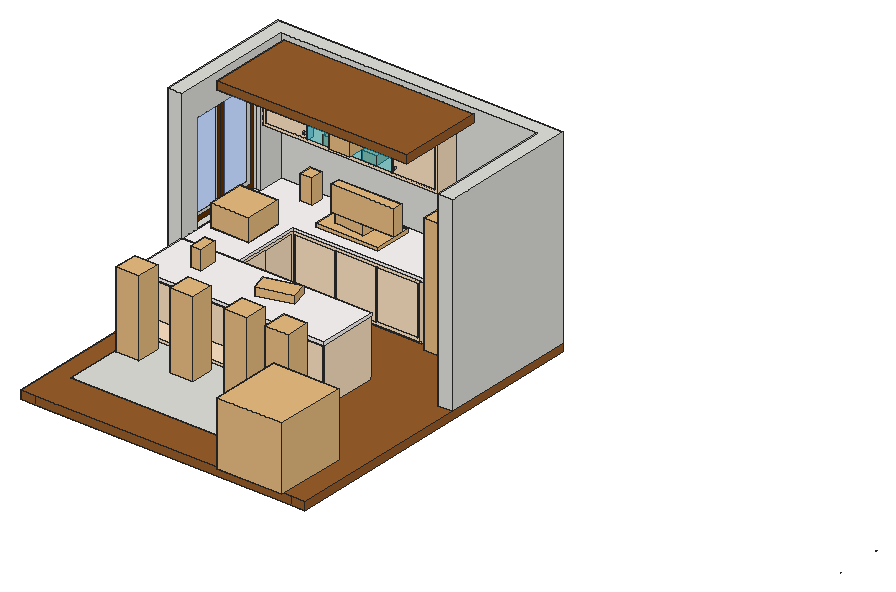
# SketchUp Ruby script. Lengths in inches.
U = 1.inch
M = Sketchup.active_model
def pt(a) = Geom::Point3d.new(a.map { |v| v * U })
def face(e, loops, mat)
  f = e.add_face(loops[0].map { |a| pt(a) })
  loops[1..].each { |l| e.add_face(l.map { |a| pt(a) }).erase! }
  f.material = f.back_material = mat if mat
  f
end
# faces: each face lists its corners as indices into pts; further lists are holes
def faces(e, pts, list, mat = nil) = list.each { |f| face(e, (f[0].is_a?(Array) ? f : [f]).map { |l| l.map { |i| pts[i] } }, mat) }
# xy, xz, yz: faces in a plane at the given z, y or x. An outline is a flat list of corners, or four numbers for a rectangle; further outlines are holes
def ring(l) = l.size == 4 ? [[l[0], l[1]], [l[2], l[1]], [l[2], l[3]], [l[0], l[3]]] : l.each_slice(2).to_a
def flat(e, list, mat, &to3) = list.each { |f| face(e, (f[0].is_a?(Array) ? f : [f]).map { |l| ring(l).map { |u, v| to3.(u, v) } }, mat) }
def xy(e, z, list, mat = nil) = flat(e, list, mat) { |x, y| [x, y, z] }
def xz(e, y, list, mat = nil) = flat(e, list, mat) { |x, z| [x, y, z] }
def yz(e, x, list, mat = nil) = flat(e, list, mat) { |y, z| [x, y, z] }
def lines(e, pts, list) = list.each { |a, b| e.add_line(pt(pts[a]), pt(pts[b])) }
# prism: a flat outline (further loops are holes) pulled along v
def prism(e, loops, v, mat = nil)
  f = face(e, loops, mat); d = Geom::Vector3d.new(v.map { |x| x * U })
  f.pushpull(f.normal.samedirection?(d) ? d.length : -d.length)
end
def box(e, o, s, mat = nil) = prism(e, [[o, [o[0] + s[0], o[1], o[2]], [o[0] + s[0], o[1] + s[1], o[2]], [o[0], o[1] + s[1], o[2]]]], [0, 0, s[2]], mat)
def at(x, y, z, deg = 0) = Geom::Transformation.translation(pt([x, y, z])) * Geom::Transformation.rotation(ORIGIN, Z_AXIS, deg.degrees)
def axes(o, x, y, z) = Geom::Transformation.new([*x, 0, *y, 0, *z, 0, *pt(o).to_a, 1])
def part(name) = M.definitions.add(name)
# library, detail: a bought-in or finely detailed component or shape, given as its bounding box
def library(name, o, s) = part(name).tap { |d| box(d.entities, o, s) }
def detail(e, o, s) = box(e.add_group.entities, o, s)
def put(e, d, t, mat = nil) = e.add_instance(d, t).tap { |i| i.material = mat if mat }
def group(e, t, mat = nil) = e.add_group.tap { |g| g.transformation = t; g.material = mat if mat }.entities
root = M.entities
M.materials.add("[0010_Snow]").color = [255, 250, 250]
M.materials.add("[0012_Bisque]").color = [255, 228, 196]
M.materials.add("[0128_White]").color = [255, 255, 255]
M.materials.add("[Color C08]").color = [102, 51, 0]
M.materials.add("[Color M00]").color = [255, 255, 255]
M.materials.add("[Translucent Glass Blue]").color = [100, 149, 237]
M.materials["[Translucent Glass Blue]"].alpha = 0.5
M.materials.add("[Translucent Glass Tinted]").color = [8, 201, 241]
M.materials["[Translucent Glass Tinted]"].alpha = 0.48
M.materials.add("[Wood Floor Dark]").color = [153, 94, 42]
c1 = part("FLOOR MAT-04")
g1 = group(c1.entities,at(-0.6,-16.77,0))
box(g1,[0,16.54,0],[111.18,64.64,0.16])
c2 = library("Stove, 5 Burners",[0,0,0],[39.37,23.7,1.97])
c3 = library("SUSPENSION ANTIQUE, maisons du monde, ref 130189 prix 249€\#1",[0,0,0.12],[23.47,23.73,45.23])
c4 = library("sink",[0,0,0],[23.82,19.09,24.47])
c5 = library("Fridge",[3.98,5.58,0],[30.88,27.96,74.41])
c6 = library("Mixer",[2.53,2.84,0],[8.2,7.51,15.59])
c7 = library("Fruits",[0,0,0],[9.5,9.5,5.38])
c8 = part("Janela aluminio")
xy(c8.entities,0,[[0,0,47.24,1.57],[23.62,1.57,47.24,2.76],[0,2.76,25.98,3.9375],[0,3.9375,47.24,5.91]])
xy(c8.entities,43.31,[[0,0,47.24,1.57],[23.62,1.57,47.24,2.76],[0,2.76,0,5.91,47.24,5.91,47.24,3.9375,25.98,3.9375,25.98,2.76],[25.98,2.76,47.24,3.9375]])
xz(c8.entities,1.57,[[0,0,23.62,0,23.62,41.34,21.26,41.34,21.26,1.97,1.97,1.97,1.97,41.34,23.62,41.34,23.62,43.31,0,43.31],[[23.62,0,47.24,43.31],[25.7,1.97,45.28,41.34]]],"[Color C08]")
xz(c8.entities,2.76,[[[0,0,23.62,43.31],[2.36,2.36,21.26,40.94]],[23.62,0,25.98,43.31]])
xz(c8.entities,2.76,[[2.36,2.36,21.26,40.94]],"[Translucent Glass Blue]")
xz(c8.entities,3.9375,[[25.98,0,25.98,2.36,44.88,2.36,44.88,40.94,25.98,40.94,25.98,43.31,47.24,43.31,47.24,0]])
xz(c8.entities,3.9375,[[25.98,2.36,44.88,40.94]],"[Translucent Glass Blue]")
yz(c8.entities,0,[[0,0,1.57,43.31],[2.76,0,5.91,43.31]])
yz(c8.entities,23.62,[[1.57,0,2.76,43.31]])
yz(c8.entities,25.98,[[2.76,0,3.9375,43.31]])
yz(c8.entities,47.24,[[0,0,1.57,43.31],[1.57,0,2.76,43.31],[3.9375,0,5.91,43.31]])
c9 = library("Group\#6",[0,0,0],[14.57,14.76,48.3])
c10 = library("Groupe\#72",[0,-0.77,0],[73.65,61.56,46.84])
c11 = library("Group\#136",[0,0,0],[6.69,11.15,11.92])
c12 = library("Groupe\#28",[6.4,0.51,-0.69],[33.32,4.86,13.24])
c13 = library("knife",[-0.45,2.4,0],[118.4,11.76,4.68])
c14 = library("Group\#508",[0,-2.9,0],[130.77,64.63,29.69])
c15 = library("Group\#498",[0,0,0],[69.53,34.78,26.97])
c16 = library("Group104",[-1707.25,-54.37,766.14],[44.8125,40.17,44.34])
xy(root,0,[[431.24,109.441,431.24,109.447,431.244,109.441],[431.24,137.782,431.24,137.788,431.244,137.788]],"[0128_White]")
xy(root,3.207,[[31.8125,137.252,45,137.803],[71.891,159,72.442,166.125],[97.751,159,98.302,166.125]])
xy(root,34.418,[[31.8125,137.252,45,137.803],[71.891,159,72.442,166.125],[97.751,159,98.302,166.125]])
xy(root,75.803,[[36.976,180.5,37.528,184.1875],[63.701,180.5,64.252,207.4375],[90.425,180.5,90.977,191.25]])
xy(root,92,[[37.528,180.5,63.701,184.1875],[64.252,180.5,90.425,184.375]],"[0012_Bisque]")
xy(root,92.551,[[37.528,180.5,63.701,184.1875],[64.252,180.5,90.425,184.375]],"[0012_Bisque]")
xy(root,108.197,[[36.976,180.5,37.528,184.1875],[63.701,180.5,64.252,207.4375],[90.425,180.5,90.977,191.25]])
xz(root,116.606,[[46.582,3.207,72.768,34.418],[72.768,3.207,73.319,34.418],[73.319,3.207,99.506,34.418],[99.506,3.207,100.057,34.418],[100.057,3.207,126.795,34.418]])
xz(root,137.252,[[31.8125,3.207,45,34.418]])
xz(root,137.803,[[31.8125,3.207,44.449,34.418],[44.449,3.207,45,34.418]])
xz(root,159,[[46.582,3.207,71.891,34.418],[72.442,3.207,97.751,34.418],[98.302,3.207,124.162,34.418]],"[0012_Bisque]")
xz(root,166.125,[[71.891,3.207,72.442,34.418],[97.751,3.207,98.302,34.418]])
xz(root,180.5,[[90.425,75.803,90.977,92],[90.425,92,90.977,108.197]])
xz(root,180.5,[[10.803,75.803,36.976,108.197],[90.977,75.803,117.701,108.197]],"[0012_Bisque]")
xz(root,180.5,[[37.528,75.803,63.701,92],[64.252,75.803,90.425,92],[37.528,92.551,63.701,108.197],[64.252,92.551,90.425,108.197]],"[Translucent Glass Tinted]")
xz(root,184.1875,[[36.976,75.803,37.528,108.197]])
xz(root,184.1875,[[37.528,92,63.701,92.551]],"[0012_Bisque]")
xz(root,184.375,[[64.252,92,90.425,92.551]],"[0012_Bisque]")
xz(root,191.25,[[90.425,75.803,90.977,108.197]])
xz(root,207.4375,[[63.701,75.803,64.252,108.197]])
yz(root,31.8125,[[137.252,3.207,137.803,34.418]])
yz(root,36.976,[[180.5,75.803,184.1875,108.197]])
yz(root,37.528,[[180.5,75.803,184.1875,92],[180.5,92.551,184.1875,108.197]])
yz(root,45,[[118.188,3.207,137.252,34.418],[137.803,3.207,157.418,34.418]],"[0012_Bisque]")
yz(root,63.701,[[180.5,75.803,207.4375,75.803,207.4375,108.197,180.5,108.197,180.5,92.551,184.1875,92.551,184.1875,92,180.5,92]])
yz(root,64.252,[[180.5,75.803,180.5,92,184.375,92,184.375,92.551,180.5,92.551,180.5,108.197,207.4375,108.197,207.4375,75.803]])
yz(root,71.891,[[159,3.207,166.125,34.418]])
yz(root,72.442,[[159,3.207,166.125,34.418]])
yz(root,90.425,[[180.5,75.803,191.25,75.803,191.25,108.197,180.5,108.197,180.5,92.551,184.375,92.551,184.375,92,180.5,92]])
yz(root,90.425,[[180.5,92,184.375,92.551]],"[0012_Bisque]")
yz(root,90.977,[[180.5,75.803,191.25,108.197]])
yz(root,97.751,[[159,3.207,166.125,34.418]])
yz(root,98.302,[[159,3.207,166.125,34.418]])
p = [[431.244,109.441,0],[431.248,109.441,0],[431.227,109.425,0],[665.051,196.66,34],[665.051,196.41,34],[695.051,196.66,34],
  [695.051,196.41,34],[743.038,200.66,71],[743.038,200.66,70.921],[743.038,200.66,106],[743.051,200.66,106],[743.051,200.66,71]]
lines(root,p,[[0,1],[1,2],[3,4],[5,6],[7,8],[9,10],[7,11]])
put(root,c1,at(12.71,25.02,0))
put(root,c2,at(53.34,166.91,38))
put(root,c3,axes([66.34,178.01,89.3],[0,-0.7224,0],[0.559,0,0],[0,0,0.4988]))
put(root,c4,axes([13.4,134.04,27.5625],[1,0,0],[0,1.19,0],[0,0,1]))
put(root,c5,axes([124.47,184.79,0],[0,-0.82,0],[1,0,0],[0,0,1]))
put(root,c6,at(40.9,180.375,37.49,90))
put(root,c7,at(47.09,180.5,76.37))
put(root,c7,at(71.34,180.5,76.37))
put(root,c7,at(45.84,180.5,93.06))
g2 = group(root,at(0,116.61,0))
xy(g2,0,[[0,0,0,87.39,180,87.39,180,0,171,0,171,78.39,9,78.39,9,0]])
xy(g2,37.78,[[0,11.3125,9,62.1875]])
xy(g2,101.47,[[0,11.3125,9,62.1875]])
xy(g2,120,[[0,0,9,0,9,78.39,171,78.39,171,0,180,0,180,87.39,0,87.39]])
xz(g2,0,[[0,0,9,120],[171,0,180,120]])
xz(g2,11.3125,[[0,37.78,9,101.47]])
xz(g2,62.1875,[[0,37.78,9,101.47]])
xz(g2,78.39,[[9,0,171,120]])
xz(g2,87.39,[[0,0,180,120]])
yz(g2,0,[[[0,0,87.39,120],[11.3125,37.78,62.1875,101.47]]])
yz(g2,9,[[[0,0,78.39,120],[11.3125,37.78,62.1875,101.47]]])
yz(g2,171,[[0,0,78.39,120]])
yz(g2,180,[[0,0,87.39,120]])
put(g2,c8,axes([5.91,11.3125,37.78],[0,1.07685,0],[-1,0,0],[0,0,1.4706]))
g3 = group(root,at(0,0,-5),"[Wood Floor Dark]")
prism(g3,[[[180,204,0],[180,0,0],[171,0,0],[9,0,0],[0,0,0],[0,204,0]]],[0,0,5])
g4 = group(root,at(9,80.61,0),"[0012_Bisque]")
xy(g4,0,[[0,0,0,114.39,116.74,114.39,116.74,79.46,34.9375,79.46,34.9375,34.9375,119.375,34.9375,119.375,0]])
xy(g4,1.58,[[1.58,0,117.79,14.5625]])
xy(g4,1.625,[[34.9375,34.9375,119.375,36],[34.9375,36,36,79.46],[36,78.39,116.74,79.46]])
xy(g4,3.21,[[37.58,23.25,117.79,36],[12.25,37.58,36,76.8125],[37.58,78.39,115.16,102.14]])
xy(g4,34.42,[[1.58,0,117.79,14.5625],[37.58,23.25,117.79,36],[12.25,37.58,36,76.8125],[37.58,78.39,115.16,102.14]])
xy(g4,36,[[0,0,119.375,0,119.375,36,36,36,36,78.39,116.74,78.39,116.74,114.39,0,114.39]])
xz(g4,0,[[[0,0,119.375,36],[1.58,1.58,117.79,34.42]]])
xz(g4,14.5625,[[1.58,1.58,117.79,34.42]])
xz(g4,23.25,[[37.58,3.21,117.79,34.42]])
xz(g4,34.9375,[[34.9375,0,119.375,1.625]])
xz(g4,36,[[[36,1.625,119.375,36],[37.58,3.21,117.79,34.42]]])
xz(g4,37.58,[[12.25,3.21,36,34.42]])
xz(g4,76.8125,[[12.25,3.21,36,34.42]])
xz(g4,78.39,[[[36,1.625,116.74,36],[37.58,3.21,115.16,34.42]]])
xz(g4,79.46,[[34.9375,0,116.74,1.625]])
xz(g4,102.14,[[37.58,3.21,115.16,34.42]])
xz(g4,114.39,[[0,0,116.74,36]])
yz(g4,0,[[0,0,114.39,36]])
yz(g4,1.58,[[0,1.58,14.5625,34.42]])
yz(g4,12.25,[[37.58,3.21,76.8125,34.42]])
yz(g4,34.9375,[[34.9375,0,79.46,1.625]])
yz(g4,36,[[[36,1.625,78.39,36],[37.58,3.21,76.8125,34.42]]])
yz(g4,37.58,[[23.25,3.21,36,34.42],[78.39,3.21,102.14,34.42]])
yz(g4,115.16,[[78.39,3.21,102.14,34.42]])
yz(g4,116.74,[[79.46,0,114.39,0,114.39,36,78.39,36,78.39,1.625,79.46,1.625]])
yz(g4,117.79,[[0,1.58,14.5625,34.42],[23.25,3.21,36,34.42]])
yz(g4,119.375,[[0,0,34.9375,0,34.9375,1.625,36,1.625,36,36,0,36]])
g5 = group(root,at(9,80.61,36),"[0010_Snow]")
prism(g5,[[[36,78.39,0],[36,36,0],[0,36,0],[0,114.39,0],[119.18,114.39,0],[119.18,78.39,0]],[[5.55,75.9,0],[5.55,53.21,0],[28.24,53.21,0],[28.24,75.9,0]]],[0,0,2])
box(g5,[0,-2.0625,0],[120.0625,37.99,2])
put(root,c9,at(107.14,59.79,-0.34))
put(root,c9,at(12.58,59.79,-0.34))
put(root,c9,at(46.45,59.79,-0.34))
put(root,c9,at(80.64,59.79,-0.34))
g6 = group(root,at(9,171,74),"[0012_Bisque]")
xy(g6,0,[[0,9.5,110.5,24]])
xy(g6,1.8,[[1.8,9.5,108.7,20.9375]])
xy(g6,34.2,[[1.8,9.5,108.7,20.9375]])
xy(g6,36,[[0,9.5,110.5,24]])
xz(g6,9.5,[[[0,0,110.5,36],[1.8,1.8,108.7,34.2]]])
xz(g6,20.9375,[[1.8,1.8,108.7,34.2]])
xz(g6,24,[[0,0,110.5,36]])
yz(g6,0,[[9.5,0,24,36]])
yz(g6,1.8,[[9.5,1.8,20.9375,34.2]])
yz(g6,108.7,[[9.5,1.8,20.9375,34.2]])
yz(g6,110.5,[[9.5,0,24,36]])
g7 = group(root,at(10.88,141.8125,111.92),"[Wood Floor Dark]")
xy(g7,0,[[0,0,119.9375,53.1875]],"[Wood Floor Dark]")
xy(g7,4.8125,[[0,0,119.9375,53.1875]],"[Wood Floor Dark]")
xz(g7,0,[[0,0,119.9375,4.8125]],"[Wood Floor Dark]")
xz(g7,53.1875,[[0,0,119.9375,4.8125]])
yz(g7,0,[[0,0,53.1875,4.8125]])
yz(g7,119.9375,[[0,0,53.1875,4.8125]])
put(root,c10,axes([125.32,-0.48,0],[0.559,0,0],[0,0.7224,0],[0,0,0.86]),"[Color M00]")
put(root,c11,at(36.84,107.94,38,-180))
put(root,c12,axes([120.38,160.98,59.53],[-1.19599,0,0],[0,-1.19599,0],[0,0,1.19599]))
g8 = group(root,at(72.81,94.34,38))
put(g8,c13,axes([7.41,14.71,1.37],[0.06872,-0.08103,0],[-0.08103,-0.06872,0],[0,0,-0.10625]))
put(g8,c14,axes([0,0,0],[0.16215,0.04345,0],[-0.04345,0.16215,0],[0,0,0.16788]))
put(root,c15,axes([79.95,181.4,39.89],[-0.27134,0.02326,0],[-0.02326,-0.27134,0],[0,0,0.27233]))
put(root,c16,axes([133.125,180.84,60.29],[0.024,0,0],[0,0.024,0],[0,0,0.024]))
put(root,c16,axes([107.25,180.84,60.29],[0.024,0,0],[0,0.024,0],[0,0,0.024]))
put(root,c16,axes([101.3125,180.84,60.29],[0.024,0,0],[0,0.024,0],[0,0,0.024]))
put(root,c16,axes([102.13,180.94,75.79],[0.024,0,0],[0,0.024,0],[0,0,0.024]))
put(root,c16,axes([106.63,180.94,75.79],[0.024,0,0],[0,0.024,0],[0,0,0.024]))
put(root,c16,axes([76.125,180.84,60.29],[0.024,0,0],[0,0.024,0],[0,0,0.024]))
